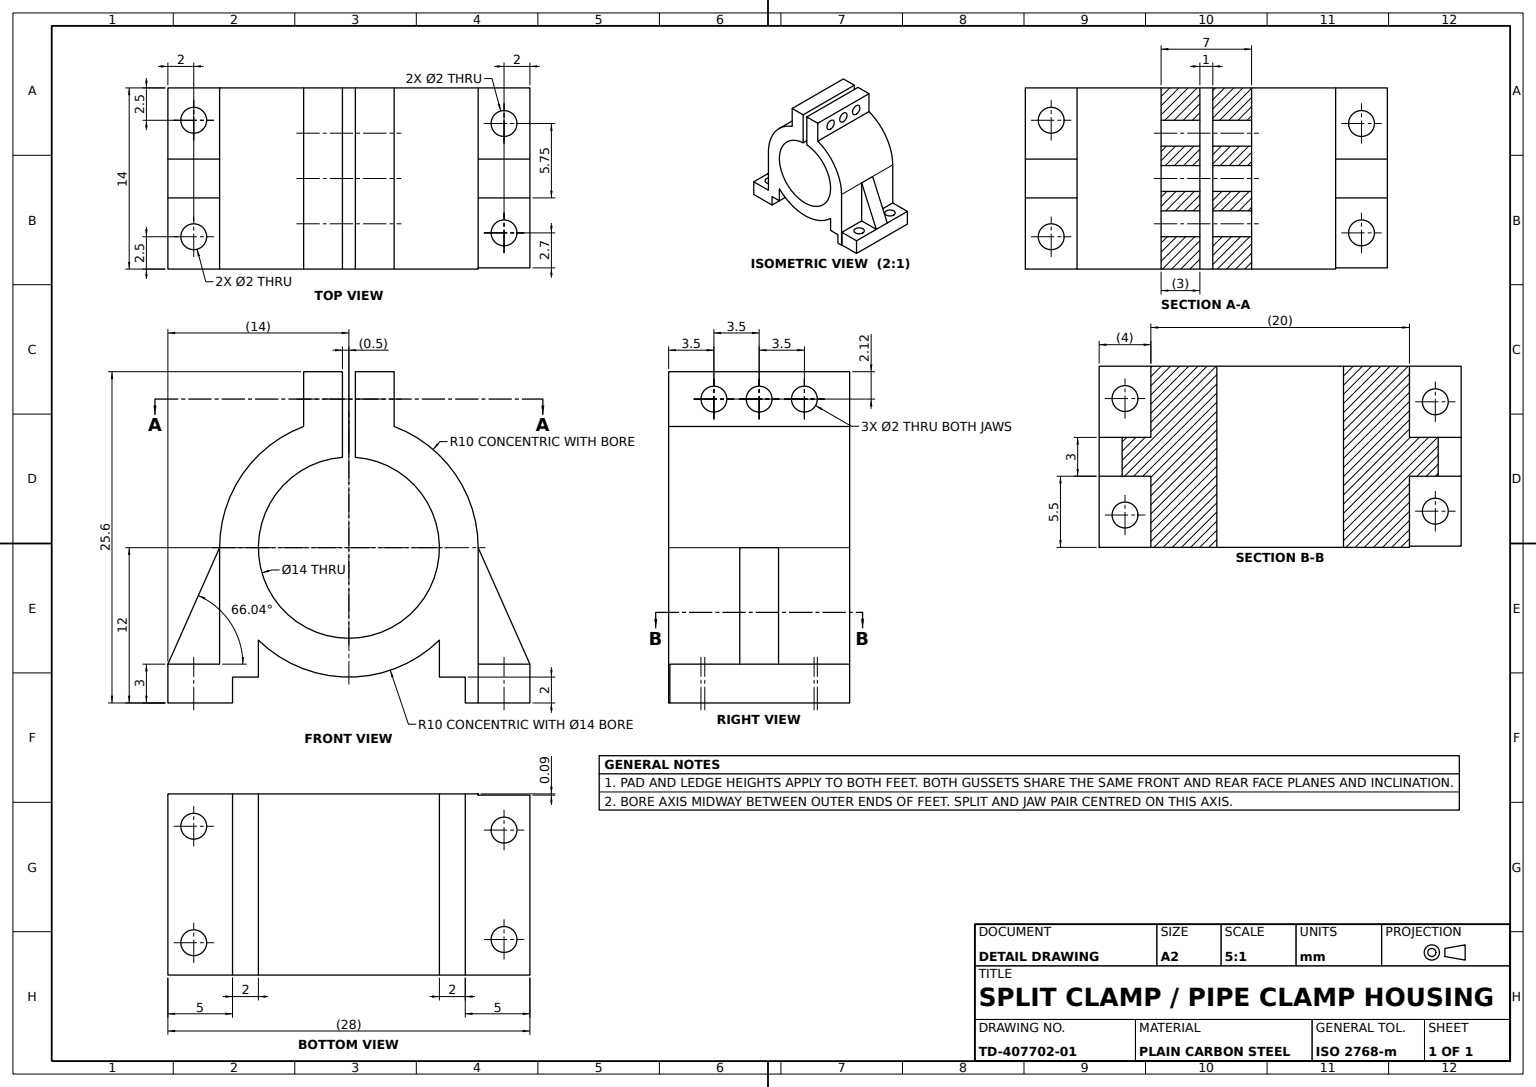
solid
v1 (10,0,0)
v2 (3.5,0,-9.367497)
e1 v1 v2 CIRCLE(AX(P(0,0,0),D(0,1,0),D(0,0,1)),10)
v3 (10,0,9)
e2 v1 v3 LINE
v4 (14,0,9)
e3 v3 v4 LINE
v5 (14,0,12)
e4 v4 v5 LINE
v6 (9,0,12)
e5 v6 v5 LINE
v7 (9,0,10)
e6 v6 v7 LINE
v8 (7,0,10)
e7 v7 v8 LINE
v9 (7,0,7.141428)
e8 v9 v8 LINE
v10 (-7,0,7.141428)
e9 v10 v9 CIRCLE(AX(P(0,0,0),D(0,1,0),D(0,0,1)),10)
v11 (-7,0,10)
e10 v10 v11 LINE
v12 (-9,0,10)
e11 v11 v12 LINE
v13 (-9,0,12)
e12 v12 v13 LINE
v14 (-14,0,12)
e13 v14 v13 LINE
v15 (-14,0,9)
e14 v15 v14 LINE
v16 (-10,0,9)
e15 v15 v16 LINE
v17 (-10,0,0)
e16 v17 v16 LINE
v18 (-3.5,0,-9.367497)
e17 v18 v17 CIRCLE(AX(P(0,0,0),D(0,1,0),D(0,0,1)),10)
v19 (-3.5,0,-13.6)
e18 v19 v18 LINE
v20 (-0.5,0,-13.6)
e19 v20 v19 LINE
v21 (-0.5,0,-6.98212)
e20 v21 v20 LINE
v22 (0.5,0,-6.98212)
e21 v21 v22 CIRCLE(AX(P(0,0,0),D(0,1,0),D(0,0,1)),7)
v23 (0.5,0,-13.6)
e22 v22 v23 LINE
v24 (3.5,0,-13.6)
e23 v24 v23 LINE
e24 v2 v24 LINE
face PLANE(AX(P(0,0,0),D(0,1,0),D(0,0,1))) rev [-e1 e2 e3 e4 -e5 e6 e7 -e8 -e9 e10 e11 e12 -e13 -e14 e15 -e16 -e17 -e18 -e19 -e20 e21 e22 -e23 -e24]
v25 (-0.5,14,-6.98212)
v26 (0.5,14,-6.98212)
e25 v25 v26 CIRCLE(AX(P(0,14,0),D(0,1,0),D(0,0,1)),7)
e26 v22 v26 LINE
e27 v21 v25 LINE
face CYL(AX(P(0,14,0),D(0,-1,0),D(0,0,-1)),7) rev [e25 -e26 -e21 e27]
v27 (3.5,7,-12.483748)
v28 (3.5,7,-10.483748)
e28 v27 v28 CIRCLE(AX(P(3.5,7,-11.483748),D(1,0,0),D(0,0,-1)),1)
e29 v28 v27 CIRCLE(AX(P(3.5,7,-11.483748),D(1,0,0),D(0,0,-1)),1)
v29 (3.5,14,-13.6)
e30 v24 v29 LINE
v30 (3.5,14,-9.367497)
e31 v29 v30 LINE
e32 v2 v30 LINE
v31 (3.5,3.5,-10.483748)
v32 (3.5,3.5,-12.483748)
e33 v31 v32 CIRCLE(AX(P(3.5,3.5,-11.483748),D(1,0,0),D(0,0,-1)),1)
e34 v32 v31 CIRCLE(AX(P(3.5,3.5,-11.483748),D(1,0,0),D(0,0,-1)),1)
v33 (3.5,10.5,-12.483748)
v34 (3.5,10.5,-10.483748)
e35 v33 v34 CIRCLE(AX(P(3.5,10.5,-11.483748),D(1,0,0),D(0,0,-1)),1)
e36 v34 v33 CIRCLE(AX(P(3.5,10.5,-11.483748),D(1,0,0),D(0,0,-1)),1)
face PLANE(AX(P(3.5,0,0),D(1,0,0),D(0,0,-1))) [-e28 -e29] [e30 e31 -e32 e24] [-e33 -e34] [-e35 -e36]
v35 (14,8.5,9)
v36 (10,8.5,0)
e37 v35 v36 LINE
v37 (10,8.5,9)
e38 v36 v37 LINE
e39 v37 v35 LINE
face PLANE(AX(P(0,8.5,0),D(0,-1,0),D(0,0,-1))) rev [e37 e38 e39]
v38 (-11,11.5,12)
v39 (-13,11.5,12)
e40 v38 v39 CIRCLE(AX(P(-12,11.5,12),D(0,0,1),D(1,0,0)),1)
e41 v39 v38 CIRCLE(AX(P(-12,11.5,12),D(0,0,1),D(1,0,0)),1)
v40 (-11,2.5,12)
v41 (-13,2.5,12)
e42 v40 v41 CIRCLE(AX(P(-12,2.5,12),D(0,0,1),D(1,0,0)),1)
e43 v41 v40 CIRCLE(AX(P(-12,2.5,12),D(0,0,1),D(1,0,0)),1)
v42 (-9,14,12)
e44 v13 v42 LINE
v43 (-14,14,12)
e45 v43 v42 LINE
e46 v43 v14 LINE
face PLANE(AX(P(0,0,12),D(0,0,1),D(1,0,0))) [-e40 -e41] [-e42 -e43] [e44 -e45 e46 e13]
v44 (-3.5,14,-9.367497)
e47 v18 v44 LINE
v45 (-3.5,14,-13.6)
e48 v45 v44 LINE
e49 v19 v45 LINE
v46 (-3.5,10.5,-12.483748)
v47 (-3.5,10.5,-10.483748)
e50 v46 v47 CIRCLE(AX(P(-3.5,10.5,-11.483748),D(-1,0,0),D(0,0,1)),1)
e51 v47 v46 CIRCLE(AX(P(-3.5,10.5,-11.483748),D(-1,0,0),D(0,0,1)),1)
v48 (-3.5,7,-10.483748)
v49 (-3.5,7,-12.483748)
e52 v48 v49 CIRCLE(AX(P(-3.5,7,-11.483748),D(-1,0,0),D(0,0,1)),1)
e53 v49 v48 CIRCLE(AX(P(-3.5,7,-11.483748),D(-1,0,0),D(0,0,1)),1)
v50 (-3.5,3.5,-12.483748)
v51 (-3.5,3.5,-10.483748)
e54 v50 v51 CIRCLE(AX(P(-3.5,3.5,-11.483748),D(-1,0,0),D(0,0,1)),1)
e55 v51 v50 CIRCLE(AX(P(-3.5,3.5,-11.483748),D(-1,0,0),D(0,0,1)),1)
face PLANE(AX(P(-3.5,0,0),D(-1,0,0),D(0,0,1))) [e47 -e48 -e49 e18] [-e50 -e51] [-e52 -e53] [-e54 -e55]
v52 (-7,14,7.141428)
e56 v10 v52 LINE
v53 (-7,14,10)
e57 v52 v53 LINE
e58 v53 v11 LINE
face PLANE(AX(P(-7,0,0),D(-1,0,0),D(0,0,1))) rev [-e10 e56 e57 e58]
v54 (0.5,10.5,-12.483748)
e59 v54 v33 LINE
v55 (0.5,10.5,-10.483748)
e60 v54 v55 CIRCLE(AX(P(0.5,10.5,-11.483748),D(-1,0,0),D(0,0,-1)),1)
e61 v55 v34 LINE
face CYL(AX(P(-29.5,10.5,-11.483748),D(1,0,0),D(0,0,-1)),1) rev [-e59 e60 e61 e36]
v56 (11,2.75,9)
v57 (13,2.75,9)
e62 v56 v57 CIRCLE(AX(P(12,2.75,9),D(0,0,-1),D(-1,0,0)),1)
v58 (13,2.75,12)
e63 v58 v57 LINE
v59 (11,2.75,12)
e64 v58 v59 CIRCLE(AX(P(12,2.75,12),D(0,0,1),D(1,0,0)),1)
e65 v59 v56 LINE
face CYL(AX(P(12,2.75,15.5),D(0,0,-1),D(-1,0,0)),1) rev [e62 -e63 e64 e65]
v60 (13,11.203154,12)
v61 (13,11.203154,9)
e66 v60 v61 LINE
v62 (11,11.203154,9)
e67 v61 v62 CIRCLE(AX(P(12,11.203154,9),D(0,0,-1),D(-1,0,0)),1)
v63 (11,11.203154,12)
e68 v63 v62 LINE
e69 v63 v60 CIRCLE(AX(P(12,11.203154,12),D(0,0,1),D(1,0,0)),1)
face CYL(AX(P(12,11.203154,15.5),D(0,0,-1),D(-1,0,0)),1) rev [e66 e67 -e68 e69]
v64 (14,5.5,9)
e70 v64 v35 LINE
v65 (14,13.906309,9)
e71 v35 v65 LINE
v66 (14,13.906309,12)
e72 v65 v66 LINE
e73 v5 v66 LINE
e74 v4 v64 LINE
face PLANE(AX(P(14,0,9),D(1,0,0),D(0,0,-1))) [e70 e71 e72 -e73 -e4 e74]
v67 (-10,8.5,9)
v68 (-10,14,9)
e75 v67 v68 LINE
v69 (-10,14,0)
e76 v69 v68 LINE
v70 (-10,8.5,0)
e77 v70 v69 LINE
e78 v67 v70 LINE
face PLANE(AX(P(-10,0,0),D(-1,0,0),D(0,0,1))) [e75 -e76 -e77 -e78]
v71 (-9,14,10)
e79 v53 v71 LINE
e80 v12 v71 LINE
face PLANE(AX(P(-7,-42,10),D(0,0,-1),D(-1,0,0))) rev [-e11 -e58 e79 -e80]
v72 (-0.5,7,-12.483748)
v73 (-0.5,7,-10.483748)
e81 v72 v73 CIRCLE(AX(P(-0.5,7,-11.483748),D(-1,0,0),D(0,0,-1)),1)
e82 v49 v72 LINE
e83 v48 v73 LINE
face CYL(AX(P(-29.5,7,-11.483748),D(1,0,0),D(0,0,-1)),1) rev [-e81 -e82 e53 e83]
e84 v55 v54 CIRCLE(AX(P(0.5,10.5,-11.483748),D(-1,0,0),D(0,0,-1)),1)
face CYL(AX(P(-29.5,10.5,-11.483748),D(1,0,0),D(0,0,-1)),1) rev [e59 e35 -e61 e84]
v74 (0.5,14,-13.6)
e85 v74 v23 LINE
e86 v29 v74 LINE
face PLANE(AX(P(3.5,14,-13.6),D(0,0,1),D(0,-1,0))) rev [e23 -e85 -e86 -e30]
v75 (0.5,7,-10.483748)
v76 (0.5,7,-12.483748)
e87 v75 v76 CIRCLE(AX(P(0.5,7,-11.483748),D(-1,0,0),D(0,0,-1)),1)
e88 v76 v27 LINE
e89 v75 v28 LINE
face CYL(AX(P(-29.5,7,-11.483748),D(1,0,0),D(0,0,-1)),1) rev [e87 e88 e28 -e89]
e90 v73 v72 CIRCLE(AX(P(-0.5,7,-11.483748),D(-1,0,0),D(0,0,-1)),1)
v77 (-0.5,3.5,-10.483748)
v78 (-0.5,3.5,-12.483748)
e91 v77 v78 CIRCLE(AX(P(-0.5,3.5,-11.483748),D(-1,0,0),D(0,0,-1)),1)
e92 v78 v77 CIRCLE(AX(P(-0.5,3.5,-11.483748),D(-1,0,0),D(0,0,-1)),1)
v79 (-0.5,14,-13.6)
e93 v25 v79 LINE
e94 v79 v20 LINE
v80 (-0.5,10.5,-10.483748)
v81 (-0.5,10.5,-12.483748)
e95 v80 v81 CIRCLE(AX(P(-0.5,10.5,-11.483748),D(-1,0,0),D(0,0,-1)),1)
e96 v81 v80 CIRCLE(AX(P(-0.5,10.5,-11.483748),D(-1,0,0),D(0,0,-1)),1)
face PLANE(AX(P(-0.5,0,0.4),D(1,0,0),D(0,0,-1))) [e81 e90] [e91 e92] [-e93 -e27 e20 -e94] [e95 e96]
face CYL(AX(P(-29.5,7,-11.483748),D(1,0,0),D(0,0,-1)),1) rev [-e83 e52 e82 -e90]
v82 (-14,8.5,9)
v83 (-14,5.5,9)
e97 v82 v83 LINE
e98 v83 v15 LINE
v84 (-14,14,9)
e99 v84 v43 LINE
e100 v84 v82 LINE
face PLANE(AX(P(-14,14,9),D(-1,0,0),D(0,-1,0))) [e97 e98 e14 -e46 -e99 e100]
v85 (-10,5.5,9)
e101 v16 v85 LINE
v86 (-10,5.5,0)
e102 v85 v86 LINE
e103 v17 v86 LINE
face PLANE(AX(P(-10,0,0),D(-1,0,0),D(0,0,1))) [e16 e101 e102 -e103]
v87 (0.5,3.5,-12.483748)
v88 (0.5,3.5,-10.483748)
e104 v87 v88 CIRCLE(AX(P(0.5,3.5,-11.483748),D(-1,0,0),D(0,0,-1)),1)
e105 v88 v87 CIRCLE(AX(P(0.5,3.5,-11.483748),D(-1,0,0),D(0,0,-1)),1)
e106 v26 v74 LINE
e107 v76 v75 CIRCLE(AX(P(0.5,7,-11.483748),D(-1,0,0),D(0,0,-1)),1)
face PLANE(AX(P(0.5,0,0.4),D(1,0,0),D(0,0,-1))) rev [-e84 -e60] [-e104 -e105] [e26 e106 e85 -e22] [-e107 -e87]
v89 (-11,11.5,9)
v90 (-13,11.5,9)
e108 v89 v90 CIRCLE(AX(P(-12,11.5,9),D(0,0,-1),D(-1,0,0)),1)
e109 v39 v90 LINE
e110 v38 v89 LINE
face CYL(AX(P(-12,11.5,19),D(0,0,-1),D(-1,0,0)),1) rev [e108 -e109 e41 e110]
v91 (10,13.906309,9)
e111 v65 v91 LINE
v92 (10,13.906309,12)
e112 v91 v92 LINE
e113 v66 v92 LINE
face PLANE(AX(P(10,13.906309,9),D(0,1,0),D(0,0,1))) [e111 e112 -e113 -e72]
v93 (-13,2.5,9)
v94 (-11,2.5,9)
e114 v93 v94 CIRCLE(AX(P(-12,2.5,9),D(0,0,-1),D(-1,0,0)),1)
e115 v40 v94 LINE
e116 v41 v93 LINE
face CYL(AX(P(-12,2.5,19),D(0,0,-1),D(-1,0,0)),1) rev [e114 -e115 e42 e116]
v95 (10,5.5,0)
e117 v1 v95 LINE
v96 (10,14,0)
e118 v96 v30 CIRCLE(AX(P(0,14,0),D(0,1,0),D(0,0,1)),10)
e119 v36 v96 LINE
e120 v95 v36 LINE
face CYL(AX(P(0,14,0),D(0,-1,0),D(0,0,-1)),10) [-e117 e1 e32 -e118 -e119 -e120]
v97 (10,14,12)
e121 v96 v97 LINE
e122 v92 v97 LINE
e123 v91 v37 LINE
face PLANE(AX(P(10,0,0),D(-1,0,0),D(0,0,1))) rev [e119 e121 -e122 -e112 e123 -e38]
e124 v46 v81 LINE
e125 v47 v80 LINE
face CYL(AX(P(-29.5,10.5,-11.483748),D(1,0,0),D(0,0,-1)),1) rev [e124 -e95 -e125 e51]
e126 v88 v31 LINE
e127 v87 v32 LINE
face CYL(AX(P(-29.5,3.5,-11.483748),D(1,0,0),D(0,0,-1)),1) rev [e126 e33 -e127 e104]
e128 v68 v84 LINE
e129 v82 v67 LINE
e130 v90 v89 CIRCLE(AX(P(-12,11.5,9),D(0,0,-1),D(-1,0,0)),1)
face PLANE(AX(P(0,0,9),D(0,0,-1),D(-1,0,0))) [-e100 -e128 -e75 -e129] [-e108 -e130]
e131 v44 v69 CIRCLE(AX(P(0,14,0),D(0,1,0),D(0,0,1)),10)
e132 v70 v86 LINE
face CYL(AX(P(0,14,0),D(0,-1,0),D(0,0,-1)),10) [e77 -e131 -e47 e17 e103 -e132]
face CYL(AX(P(-29.5,10.5,-11.483748),D(1,0,0),D(0,0,-1)),1) rev [e125 -e96 -e124 e50]
e133 v51 v77 LINE
e134 v50 v78 LINE
face CYL(AX(P(-29.5,3.5,-11.483748),D(1,0,0),D(0,0,-1)),1) rev [e133 -e92 -e134 e54]
e135 v83 v85 LINE
e136 v94 v93 CIRCLE(AX(P(-12,2.5,9),D(0,0,-1),D(-1,0,0)),1)
face PLANE(AX(P(0,0,9),D(0,0,-1),D(-1,0,0))) [-e98 e135 -e101 -e15] [-e114 -e136]
v98 (10,5.5,9)
e137 v95 v98 LINE
e138 v64 v95 LINE
e139 v98 v64 LINE
face PLANE(AX(P(0,5.5,0),D(0,-1,0),D(0,0,-1))) [-e137 -e138 -e139]
e140 v62 v61 CIRCLE(AX(P(12,11.203154,9),D(0,0,-1),D(-1,0,0)),1)
face PLANE(AX(P(0,0,9),D(0,0,-1),D(-1,0,0))) [-e123 -e111 -e71 -e39] [-e140 -e67]
v99 (9,14,10)
v100 (7,14,10)
e141 v99 v100 LINE
e142 v100 v8 LINE
e143 v7 v99 LINE
face PLANE(AX(P(9,-78,10),D(0,0,-1),D(-1,0,0))) rev [e141 e142 -e7 e143]
e144 v79 v45 LINE
face PLANE(AX(P(3.5,14,-13.6),D(0,0,1),D(0,-1,0))) rev [-e144 e94 e19 e49]
v101 (7,14,7.141428)
e145 v9 v101 LINE
e146 v52 v101 CIRCLE(AX(P(0,14,0),D(0,1,0),D(0,0,1)),10)
face CYL(AX(P(0,14,0),D(0,-1,0),D(0,0,-1)),10) [-e56 e9 e145 -e146]
v102 (9,14,12)
e147 v6 v102 LINE
e148 v102 v97 LINE
e149 v59 v58 CIRCLE(AX(P(12,2.75,12),D(0,0,1),D(1,0,0)),1)
e150 v60 v63 CIRCLE(AX(P(12,11.203154,12),D(0,0,1),D(1,0,0)),1)
face PLANE(AX(P(0,0,12),D(0,0,1),D(1,0,0))) [-e147 e5 e73 e113 e122 -e148] [-e64 -e149] [-e69 -e150]
e151 v101 v100 LINE
e152 v102 v99 LINE
e153 v71 v42 LINE
face PLANE(AX(P(0,14,0),D(0,1,0),D(0,0,1))) [e151 -e141 -e152 e148 -e121 e118 -e31 e86 -e106 -e25 e93 e144 e48 e131 e76 e128 e99 e45 -e153 -e79 -e57 e146]
face CYL(AX(P(-12,11.5,19),D(0,0,-1),D(-1,0,0)),1) rev [-e110 e40 e109 e130]
face PLANE(AX(P(-9,-42,12),D(-1,0,0),D(0,0,1))) rev [-e12 e80 e153 -e44]
face PLANE(AX(P(9,-78,12),D(1,0,0),D(0,0,-1))) rev [-e6 e147 e152 -e143]
face CYL(AX(P(-29.5,7,-11.483748),D(1,0,0),D(0,0,-1)),1) rev [e107 e89 e29 -e88]
e154 v98 v3 LINE
face PLANE(AX(P(10,0,0),D(-1,0,0),D(0,0,1))) rev [e137 e154 -e2 e117]
e155 v57 v56 CIRCLE(AX(P(12,2.75,9),D(0,0,-1),D(-1,0,0)),1)
face PLANE(AX(P(0,0,9),D(0,0,-1),D(-1,0,0))) [-e3 -e154 e139 -e74] [-e155 -e62]
face CYL(AX(P(-29.5,3.5,-11.483748),D(1,0,0),D(0,0,-1)),1) rev [e34 -e126 e105 e127]
face PLANE(AX(P(7,0,0),D(-1,0,0),D(0,0,1))) [-e142 -e151 -e145 e8]
e156 v70 v82 LINE
face PLANE(AX(P(0,8.5,0),D(0,-1,0),D(0,0,-1))) rev [e78 e156 e129]
face CYL(AX(P(12,2.75,15.5),D(0,0,-1),D(-1,0,0)),1) rev [e149 e63 e155 -e65]
face CYL(AX(P(-29.5,3.5,-11.483748),D(1,0,0),D(0,0,-1)),1) rev [e134 -e91 -e133 e55]
face PLANE(AX(P(14,5.5,9),D(0.913811549,0,-0.406138466),D(-0.406138466,0,-0.913811549))) [-e70 e138 e120 -e37]
face CYL(AX(P(-12,2.5,19),D(0,0,-1),D(-1,0,0)),1) rev [e115 e136 -e116 e43]
e157 v86 v83 LINE
face PLANE(AX(P(0,5.5,0),D(0,-1,0),D(0,0,-1))) [-e135 -e157 -e102]
face CYL(AX(P(12,11.203154,15.5),D(0,0,-1),D(-1,0,0)),1) rev [e150 e68 e140 -e66]
face PLANE(AX(P(-10,8.5,0),D(0.913811549,0,0.406138466),D(0.406138466,0,-0.913811549))) rev [e157 -e97 -e156 e132]
